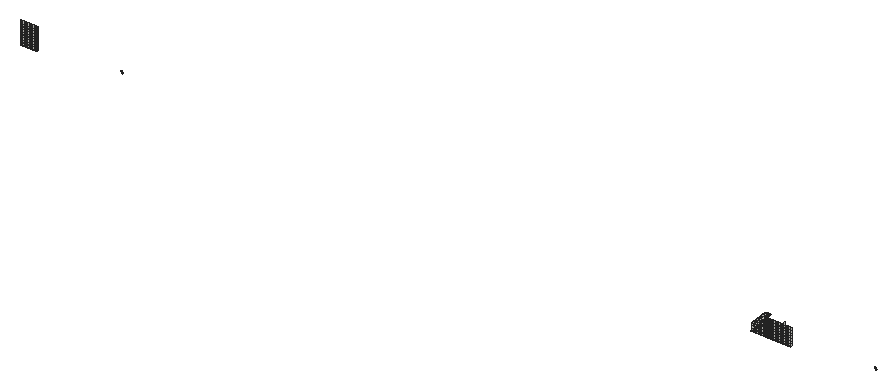
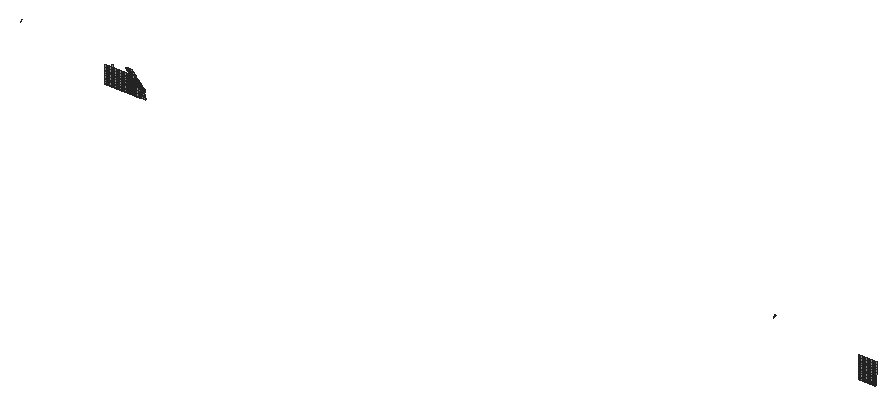
# SketchUp Ruby script. Lengths in inches.
U = 1.inch
M = Sketchup.active_model
def pt(a) = Geom::Point3d.new(a.map { |v| v * U })
def face(e, loops, mat)
  f = e.add_face(loops[0].map { |a| pt(a) })
  loops[1..].each { |l| e.add_face(l.map { |a| pt(a) }).erase! }
  f.material = f.back_material = mat if mat
  f
end
# faces: each face lists its corners as indices into pts; further lists are holes
def faces(e, pts, list, mat = nil) = list.each { |f| face(e, (f[0].is_a?(Array) ? f : [f]).map { |l| l.map { |i| pts[i] } }, mat) }
# xy, xz, yz: faces in a plane at the given z, y or x. An outline is a flat list of corners, or four numbers for a rectangle; further outlines are holes
def ring(l) = l.size == 4 ? [[l[0], l[1]], [l[2], l[1]], [l[2], l[3]], [l[0], l[3]]] : l.each_slice(2).to_a
def flat(e, list, mat, &to3) = list.each { |f| face(e, (f[0].is_a?(Array) ? f : [f]).map { |l| ring(l).map { |u, v| to3.(u, v) } }, mat) }
def xy(e, z, list, mat = nil) = flat(e, list, mat) { |x, y| [x, y, z] }
def xz(e, y, list, mat = nil) = flat(e, list, mat) { |x, z| [x, y, z] }
def yz(e, x, list, mat = nil) = flat(e, list, mat) { |y, z| [x, y, z] }
def lines(e, pts, list) = list.each { |a, b| e.add_line(pt(pts[a]), pt(pts[b])) }
# prism: a flat outline (further loops are holes) pulled along v
def prism(e, loops, v, mat = nil)
  f = face(e, loops, mat); d = Geom::Vector3d.new(v.map { |x| x * U })
  f.pushpull(f.normal.samedirection?(d) ? d.length : -d.length)
end
def box(e, o, s, mat = nil) = prism(e, [[o, [o[0] + s[0], o[1], o[2]], [o[0] + s[0], o[1] + s[1], o[2]], [o[0], o[1] + s[1], o[2]]]], [0, 0, s[2]], mat)
def at(x, y, z, deg = 0) = Geom::Transformation.translation(pt([x, y, z])) * Geom::Transformation.rotation(ORIGIN, Z_AXIS, deg.degrees)
def axes(o, x, y, z) = Geom::Transformation.new([*x, 0, *y, 0, *z, 0, *pt(o).to_a, 1])
def part(name) = M.definitions.add(name)
# library, detail: a bought-in or finely detailed component or shape, given as its bounding box
def library(name, o, s) = part(name).tap { |d| box(d.entities, o, s) }
def detail(e, o, s) = box(e.add_group.entities, o, s)
def put(e, d, t, mat = nil) = e.add_instance(d, t).tap { |i| i.material = mat if mat }
def group(e, t, mat = nil) = e.add_group.tap { |g| g.transformation = t; g.material = mat if mat }.entities
root = M.entities
M.materials.add("[Color M06]").color = [79, 71, 84]
xy(root,341.65,[[1366.25,480.14,1368.57,480.77],[1369.17,480.14,1371.48,480.77],[1372.08,480.14,1374.39,480.77],[1374.99,480.14,1377.3,480.77],[1377.9,480.14,1380.22,480.77],
  [1380.81,480.14,1383.13,480.77],[1383.73,480.14,1386.04,480.77],[2225.11,480.14,2225.91,480.77],[2226.51,480.14,2228.82,480.77],[2229.42,480.14,2231.73,480.77],
  [2232.33,480.14,2234.65,480.77],[2235.25,480.14,2237.56,480.77],[2238.16,480.14,2240.47,480.77],[2241.07,480.14,2243.38,480.77],[2243.98,480.14,2246.29,480.77],
  [2246.89,480.14,2249.21,480.77],[2249.81,480.14,2252.12,480.77],[2252.72,480.14,2255.03,480.77],[2255.63,480.14,2257.94,480.77],[2258.54,480.14,2260.86,480.77],
  [2261.45,480.14,2263.77,480.77],[2264.37,480.14,2266.68,480.77],[2267.28,480.14,2269.59,480.77],[2270.19,480.14,2272.5,480.77]])
xy(root,342.15,[[1366.25,480.14,1368.57,480.77],[1369.17,480.14,1371.48,480.77],[1372.08,480.14,1374.39,480.77],[1374.99,480.14,1377.3,480.77],[1377.9,480.14,1380.22,480.77],
  [1380.81,480.14,1383.13,480.77],[1383.73,480.14,1386.04,480.77],[2226.51,480.14,2228.82,480.77],[2229.42,480.14,2231.73,480.77],[2232.33,480.14,2234.65,480.77],
  [2235.25,480.14,2237.56,480.77],[2238.16,480.14,2240.47,480.77],[2241.07,480.14,2243.38,480.77],[2243.98,480.14,2246.29,480.77],[2246.89,480.14,2249.21,480.77],
  [2249.81,480.14,2252.12,480.77],[2252.72,480.14,2255.03,480.77],[2255.63,480.14,2257.94,480.77],[2258.54,480.14,2260.86,480.77],[2261.45,480.14,2263.77,480.77],
  [2264.37,480.14,2266.68,480.77],[2267.28,480.14,2269.59,480.77],[2270.19,480.14,2272.5,480.77]])
xy(root,344.46,[[1366.25,480.14,1368.57,480.77],[1369.17,480.14,1371.48,480.77],[1372.08,480.14,1374.39,480.77],[1374.99,480.14,1377.3,480.77],[1377.9,480.14,1380.22,480.77],
  [1380.81,480.14,1383.13,480.77],[2227.75,480.14,2228.82,480.77],[2229.42,480.14,2231.73,480.77],[2232.33,480.14,2234.65,480.77],[2235.25,480.14,2237.56,480.77],
  [2238.16,480.14,2240.47,480.77],[2241.07,480.14,2243.38,480.77],[2243.98,480.14,2246.29,480.77],[2246.89,480.14,2249.21,480.77],[2249.81,480.14,2252.12,480.77],
  [2252.72,480.14,2255.03,480.77],[2255.63,480.14,2257.94,480.77],[2258.54,480.14,2260.86,480.77],[2261.45,480.14,2263.77,480.77],[2264.37,480.14,2266.68,480.77],
  [2267.28,480.14,2269.59,480.77]])
xy(root,344.96,[[1366.25,480.14,1368.57,480.77],[1369.17,480.14,1371.48,480.77],[1372.08,480.14,1374.39,480.77],[1374.99,480.14,1377.3,480.77],[1377.9,480.14,1380.22,480.77],
  [1380.81,480.14,1383.13,480.77],[1383.73,480.14,1386.04,480.77],[2229.42,480.14,2231.73,480.77],[2232.33,480.14,2234.65,480.77],[2235.25,480.14,2237.56,480.77],
  [2238.16,480.14,2240.47,480.77],[2241.07,480.14,2243.38,480.77],[2243.98,480.14,2246.29,480.77],[2246.89,480.14,2249.21,480.77],[2249.81,480.14,2252.12,480.77],
  [2252.72,480.14,2255.03,480.77],[2255.63,480.14,2257.94,480.77],[2258.54,480.14,2260.86,480.77],[2261.45,480.14,2263.77,480.77],[2264.37,480.14,2266.68,480.77],
  [2267.28,480.14,2269.59,480.77],[2270.19,480.14,2272.5,480.77]])
xy(root,347.27,[[1366.25,480.14,1368.57,480.77],[1369.17,480.14,1371.48,480.77],[1372.08,480.14,1374.39,480.77],[1374.99,480.14,1377.3,480.77],[1377.9,480.14,1380.22,480.77],
  [1380.81,480.14,1383.13,480.77],[1383.73,480.14,1386.04,480.77],[2230.38,480.14,2231.73,480.77],[2232.33,480.14,2234.65,480.77],[2235.25,480.14,2237.56,480.77],
  [2238.16,480.14,2240.47,480.77],[2241.07,480.14,2243.38,480.77],[2243.98,480.14,2246.29,480.77],[2246.89,480.14,2249.21,480.77],[2249.81,480.14,2252.12,480.77],
  [2252.72,480.14,2255.03,480.77],[2255.63,480.14,2257.94,480.77],[2258.54,480.14,2260.86,480.77],[2261.45,480.14,2263.77,480.77],[2264.37,480.14,2266.68,480.77],
  [2267.28,480.14,2269.59,480.77],[2270.19,480.14,2272.5,480.77]])
xy(root,347.77,[[1366.25,480.14,1368.57,480.77],[1369.17,480.14,1371.48,480.77],[1372.08,480.14,1374.39,480.77],[1374.99,480.14,1377.3,480.77],[1377.9,480.14,1380.22,480.77],
  [1380.81,480.14,1383.13,480.77],[1383.73,480.14,1386.04,480.77],[2232.33,480.14,2234.65,480.77],[2235.25,480.14,2237.56,480.77],[2238.16,480.14,2240.47,480.77],
  [2241.07,480.14,2243.38,480.77],[2243.98,480.14,2246.29,480.77],[2246.89,480.14,2249.21,480.77],[2249.81,480.14,2252.12,480.77],[2252.72,480.14,2255.03,480.77],
  [2255.63,480.14,2257.94,480.77],[2258.54,480.14,2260.86,480.77],[2261.45,480.14,2263.77,480.77],[2264.37,480.14,2266.68,480.77],[2267.28,480.14,2269.59,480.77],
  [2270.19,480.14,2272.5,480.77]])
xy(root,350.09,[[1366.25,480.14,1368.57,480.77],[1369.17,480.14,1371.48,480.77],[1372.08,480.14,1374.39,480.77],[1374.99,480.14,1377.3,480.77],[1377.9,480.14,1380.22,480.77],
  [1380.81,480.14,1383.13,480.77],[1383.73,480.14,1386.04,480.77],[2233.02,480.14,2234.65,480.77],[2235.25,480.14,2237.56,480.77],[2238.16,480.14,2240.47,480.77],
  [2241.07,480.14,2243.38,480.77],[2243.98,480.14,2246.29,480.77],[2246.89,480.14,2249.21,480.77],[2249.81,480.14,2252.12,480.77],[2252.72,480.14,2255.03,480.77],
  [2255.63,480.14,2257.94,480.77],[2258.54,480.14,2260.86,480.77],[2261.45,480.14,2263.77,480.77],[2264.37,480.14,2266.68,480.77],[2267.28,480.14,2269.59,480.77],
  [2270.19,480.14,2272.5,480.77]])
xy(root,350.59,[[1366.25,480.14,1368.57,480.77],[1369.17,480.14,1371.48,480.77],[1372.08,480.14,1374.39,480.77],[1374.99,480.14,1377.3,480.77],[1377.9,480.14,1380.22,480.77],
  [1380.81,480.14,1383.13,480.77],[1383.73,480.14,1386.04,480.77],[2235.25,480.14,2237.56,480.77],[2238.16,480.14,2240.47,480.77],[2241.07,480.14,2243.38,480.77],
  [2243.98,480.14,2246.29,480.77],[2246.89,480.14,2249.21,480.77],[2249.81,480.14,2252.12,480.77],[2252.72,480.14,2255.03,480.77],[2255.63,480.14,2257.94,480.77],
  [2258.54,480.14,2260.86,480.77],[2261.45,480.14,2263.77,480.77],[2264.37,480.14,2266.68,480.77],[2267.28,480.14,2269.59,480.77],[2270.19,480.14,2272.5,480.77]])
xy(root,352.9,[[1366.25,480.14,1368.57,480.77],[1369.17,480.14,1371.48,480.77],[1372.08,480.14,1374.39,480.77],[1374.99,480.14,1377.3,480.77],[1377.9,480.14,1380.22,480.77],
  [1380.81,480.14,1383.13,480.77],[1383.73,480.14,1386.04,480.77],[2235.65,480.14,2237.56,480.77],[2238.16,480.14,2240.47,480.77],[2241.07,480.14,2243.38,480.77],
  [2243.98,480.14,2246.29,480.77],[2246.89,480.14,2249.21,480.77],[2249.81,480.14,2252.12,480.77],[2252.72,480.14,2255.03,480.77],[2255.63,480.14,2257.94,480.77],
  [2258.54,480.14,2260.86,480.77],[2261.45,480.14,2263.77,480.77],[2264.37,480.14,2266.68,480.77],[2267.28,480.14,2269.59,480.77],[2270.19,480.14,2272.5,480.77]])
xy(root,353.4,[[1366.25,480.14,1368.57,480.77],[1369.17,480.14,1371.48,480.77],[1372.08,480.14,1374.39,480.77],[1374.99,480.14,1377.3,480.77],[1377.9,480.14,1380.22,480.77],
  [1380.81,480.14,1383.13,480.77],[1383.73,480.14,1386.04,480.77],[2236.12,480.14,2237.56,480.77],[2238.16,480.14,2240.47,480.77],[2241.07,480.14,2243.38,480.77],
  [2243.98,480.14,2246.29,480.77],[2246.89,480.14,2249.21,480.77],[2249.81,480.14,2252.12,480.77],[2252.72,480.14,2255.03,480.77],[2255.63,480.14,2257.94,480.77],
  [2258.54,480.14,2260.86,480.77],[2261.45,480.14,2263.77,480.77],[2264.37,480.14,2266.68,480.77],[2267.28,480.14,2269.59,480.77],[2270.19,480.14,2272.5,480.77]])
xy(root,355.71,[[1366.25,480.14,1368.57,480.77],[1369.17,480.14,1371.48,480.77],[1372.08,480.14,1374.39,480.77],[1374.99,480.14,1377.3,480.77],[1377.9,480.14,1380.22,480.77],
  [1380.81,480.14,1383.13,480.77],[1383.73,480.14,1386.04,480.77],[2238.29,480.14,2240.47,480.77],[2241.07,480.14,2243.38,480.77],[2243.98,480.14,2246.29,480.77],
  [2246.89,480.14,2249.21,480.77],[2249.81,480.14,2252.12,480.77],[2252.72,480.14,2255.03,480.77],[2255.63,480.14,2257.94,480.77],[2258.54,480.14,2260.86,480.77],
  [2261.45,480.14,2263.77,480.77],[2264.37,480.14,2266.68,480.77],[2267.28,480.14,2269.59,480.77],[2270.19,480.14,2272.5,480.77]])
xy(root,356.21,[[1366.25,480.14,1368.57,480.77],[1369.17,480.14,1371.48,480.77],[1372.08,480.14,1374.39,480.77],[1374.99,480.14,1377.3,480.77],[1377.9,480.14,1380.22,480.77],
  [1380.81,480.14,1383.13,480.77],[1383.73,480.14,1386.04,480.77],[2238.76,480.14,2240.47,480.77],[2241.07,480.14,2243.38,480.77],[2243.98,480.14,2246.29,480.77],
  [2246.89,480.14,2249.21,480.77],[2249.81,480.14,2252.12,480.77],[2252.72,480.14,2255.03,480.77],[2255.63,480.14,2257.94,480.77],[2258.54,480.14,2260.86,480.77],
  [2261.45,480.14,2263.77,480.77],[2264.37,480.14,2266.68,480.77],[2267.28,480.14,2269.59,480.77],[2270.19,480.14,2272.5,480.77]])
xy(root,358.52,[[1366.25,480.14,1368.57,480.77],[1369.17,480.14,1371.48,480.77],[1372.08,480.14,1374.39,480.77],[1374.99,480.14,1377.3,480.77],[1377.9,480.14,1380.22,480.77],
  [1380.81,480.14,1383.13,480.77],[1383.73,480.14,1386.04,480.77],[2241.07,480.14,2243.38,480.77],[2243.98,480.14,2246.29,480.77],[2246.89,480.14,2249.21,480.77],
  [2249.81,480.14,2252.12,480.77],[2252.72,480.14,2255.03,480.77],[2255.63,480.14,2257.94,480.77],[2258.54,480.14,2260.86,480.77],[2261.45,480.14,2263.77,480.77],
  [2264.37,480.14,2266.68,480.77],[2267.28,480.14,2269.59,480.77],[2270.19,480.14,2272.5,480.77]])
xy(root,359.02,[[1366.25,480.14,1368.57,480.77],[1369.17,480.14,1371.48,480.77],[1372.08,480.14,1374.39,480.77],[1374.99,480.14,1377.3,480.77],[1377.9,480.14,1380.22,480.77],
  [1380.81,480.14,1383.13,480.77],[1383.73,480.14,1386.04,480.77],[2241.4,480.14,2243.38,480.77],[2243.98,480.14,2246.29,480.77],[2246.89,480.14,2249.21,480.77],
  [2249.81,480.14,2252.12,480.77],[2252.72,480.14,2255.03,480.77],[2255.63,480.14,2257.94,480.77],[2258.54,480.14,2260.86,480.77],[2261.45,480.14,2263.77,480.77],
  [2264.37,480.14,2266.68,480.77],[2267.28,480.14,2269.59,480.77],[2270.19,480.14,2272.5,480.77]])
xy(root,361.34,[[1366.25,480.14,1368.57,480.77],[1369.17,480.14,1371.48,480.77],[1372.08,480.14,1374.39,480.77],[1374.99,480.14,1377.3,480.77],[1377.9,480.14,1380.22,480.77],
  [1380.81,480.14,1383.13,480.77],[1383.73,480.14,1386.04,480.77],[2243.98,480.14,2246.29,480.77],[2246.89,480.14,2249.21,480.77],[2249.81,480.14,2252.12,480.77],
  [2252.72,480.14,2255.03,480.77],[2255.63,480.14,2257.94,480.77],[2258.54,480.14,2260.86,480.77],[2261.45,480.14,2263.77,480.77],[2264.37,480.14,2266.68,480.77],
  [2267.28,480.14,2269.59,480.77],[2270.19,480.14,2272.5,480.77]])
xy(root,361.84,[[1366.25,480.14,1368.57,480.77],[1369.17,480.14,1371.48,480.77],[1372.08,480.14,1374.39,480.77],[1374.99,480.14,1377.3,480.77],[1377.9,480.14,1380.22,480.77],
  [1380.81,480.14,1383.13,480.77],[1383.73,480.14,1386.04,480.77]])
xy(root,364.15,[[1366.25,480.14,1368.57,480.77],[1369.17,480.14,1371.48,480.77],[1372.08,480.14,1374.39,480.77],[1374.99,480.14,1377.3,480.77],[1377.9,480.14,1380.22,480.77],
  [1380.81,480.14,1383.13,480.77],[1383.73,480.14,1386.04,480.77]])
xy(root,364.65,[[1366.25,480.14,1368.57,480.77],[1369.17,480.14,1371.48,480.77],[1372.08,480.14,1374.39,480.77],[1374.99,480.14,1377.3,480.77],[1377.9,480.14,1380.22,480.77],
  [1380.81,480.14,1383.13,480.77],[1383.73,480.14,1386.04,480.77]])
xz(root,467.1875,[[1496.3,361.83,1496.67,362.07,1494.98,364.71,1494.61,364.48],[2382.77,361.83,2383.14,362.07,2381.44,364.71,2381.07,364.48]],"[Color M06]")
xz(root,480.14,[[2226.51,343.14,2227.75,344.46,2226.51,344.46],[2226.51,344.96,2228.21,344.96,2228.82,345.61,2228.82,347.27,2227.75,347.27,2226.51,345.96],[2228.21,344.96,2228.82,344.96,2228.82,345.61],[2229.42,346.25,2230.38,347.27,2229.42,347.27],[2226.51,347.77,2226.52,347.77,2228.69,350.09,2227.75,350.09,2226.51,348.77],
  [2226.52,347.77,2228.21,347.77,2228.82,348.42,2228.82,350.09,2228.69,350.09],[2229.42,347.77,2230.85,347.77,2231.73,348.72,2231.73,350.09,2230.38,350.09,2229.42,349.0625],[2230.85,347.77,2231.73,347.77,2231.73,348.72],[2232.33,349.36,2233.02,350.09,2232.33,350.09],[2226.52,350.59,2226.57,350.59,2228.75,352.9,2228.69,352.9],
  [2226.57,350.59,2228.21,350.59,2228.82,351.24,2228.82,352.9,2228.75,352.9],[2228.21,350.59,2228.82,350.59,2228.82,351.24],[2229.42,350.59,2230.85,350.59,2231.73,351.53,2231.73,352.9,2231.34,352.9,2229.42,350.86],[2232.33,350.59,2233.49,350.59,2234.65,351.82,2234.65,352.9,2233.02,352.9,2232.33,352.17],[2233.49,350.59,2234.65,350.59,2234.65,351.82],
  [2229.42,350.86,2231.34,352.9,2230.38,352.9,2229.42,351.875],[2235.25,352.46,2235.65,352.9,2235.25,352.9],[2229.42,353.4,2230.85,353.4,2231.73,354.34,2231.73,355.71,2231.4,355.71,2229.42,353.62],[2230.85,353.4,2231.73,353.4,2231.73,354.34],[2232.33,353.4,2233.49,353.4,2234.65,354.64,2234.65,355.71,2233.99,355.71,2232.33,353.95],
  [2235.25,353.4,2236.12,353.4,2237.56,354.93,2237.56,355.71,2235.65,355.71,2235.25,355.28],[2229.42,353.62,2231.4,355.71,2231.34,355.71,2229.42,353.67],[2232.33,353.95,2233.99,355.71,2233.02,355.71,2232.33,354.98],[2238.16,355.57,2238.29,355.71,2238.16,355.71],[2232.33,356.21,2233.49,356.21,2234.65,357.45,2234.65,358.52,2234.04,358.52,2232.33,356.71],
  [2234.46,356.21,2234.65,356.21,2234.65,356.41],[2235.25,356.21,2236.12,356.21,2237.56,357.74,2237.56,358.52,2236.64,358.52,2235.25,357.05],[2238.16,356.21,2238.76,356.21,2240.47,358.04,2240.47,358.52,2238.29,358.52,2238.16,358.38],[2232.33,356.71,2234.04,358.52,2233.99,358.52,2232.33,356.77],[2235.25,357.05,2236.64,358.52,2235.65,358.52,2235.25,358.09],
  [2238.16,358.38,2238.29,358.52,2238.16,358.52],[2234.51,359.02,2234.65,359.02,2234.65,359.17],[2235.25,359.02,2236.12,359.02,2237.56,360.56,2237.56,361.34,2236.69,361.34,2235.25,359.8],[2237.11,359.02,2237.56,359.02,2237.56,359.5],[2238.16,359.02,2240.47,359.02,2240.47,361.34,2239.28,361.34,2238.16,360.14],
  [2241.07,359.02,2241.4,359.02,2243.38,361.14,2243.38,361.34,2241.07,361.34],[2235.25,359.8,2236.69,361.34,2236.64,361.34,2235.25,359.86],[2238.16,361.2,2238.29,361.34,2238.16,361.34],[2237.16,361.84,2237.56,361.84,2237.56,362.26],[2238.16,361.84,2239.75,361.84,2240.47,362.6,2240.47,364.15,2239.34,364.15,2238.16,362.9],
  [2239.75,361.84,2240.47,361.84,2240.47,362.6],[2241.07,361.84,2241.4,361.84,2243.38,363.96,2243.38,364.15,2241.93,364.15,2241.07,363.23],[2241.4,361.84,2243.38,361.84,2243.38,363.96],[2241.07,363.23,2241.93,364.15,2241.07,364.15],[2239.81,364.65,2240.47,364.65,2240.47,365.35],
  [2241.07,364.65,2241.4,364.65,2243.38,366.77,2243.38,366.96,2241.99,366.96,2241.07,365.99],[2241.4,364.65,2242.4,364.65,2243.38,365.69,2243.38,366.77],[2242.4,364.65,2243.38,364.65,2243.38,365.69],[2243.98,364.65,2244.03,364.65,2246.2,366.96,2244.58,366.96,2243.98,366.33],[2244.03,364.65,2246.29,364.65,2246.29,366.96,2246.2,366.96]])
xz(root,480.14,[[2243.98,361.84,2244.03,361.84,2246.2,364.15,2243.98,364.15],[2246.89,364.89,2248.83,366.96,2246.89,366.96]],"[Color M06]")
yz(root,1365.65,[[480.14,353.4,480.77,355.71],[480.14,356.21,480.77,358.52],[480.14,359.02,480.77,361.34],[480.14,361.84,480.77,364.15],[480.14,364.65,480.77,366.96]])
yz(root,1366.25,[[480.14,342.15,480.77,344.46],[480.14,344.96,480.77,347.27],[480.14,347.77,480.77,350.09],[480.14,350.59,480.77,352.9],[480.14,353.4,480.77,355.71],
  [480.14,356.21,480.77,358.52],[480.14,359.02,480.77,361.34],[480.14,361.84,480.77,364.15],[480.14,364.65,480.77,366.96]])
yz(root,1368.57,[[480.14,342.15,480.77,344.46],[480.14,344.96,480.77,347.27],[480.14,347.77,480.77,350.09],[480.14,350.59,480.77,352.9],[480.14,353.4,480.77,355.71],
  [480.14,356.21,480.77,358.52],[480.14,359.02,480.77,361.34],[480.14,361.84,480.77,364.15],[480.14,364.65,480.77,366.96]])
yz(root,1369.17,[[480.14,342.15,480.77,344.46],[480.14,344.96,480.77,347.27],[480.14,347.77,480.77,350.09],[480.14,350.59,480.77,352.9],[480.14,353.4,480.77,355.71],
  [480.14,356.21,480.77,358.52],[480.14,359.02,480.77,361.34],[480.14,361.84,480.77,364.15],[480.14,364.65,480.77,366.96]])
yz(root,1371.48,[[480.14,342.15,480.77,344.46],[480.14,344.96,480.77,347.27],[480.14,347.77,480.77,350.09],[480.14,350.59,480.77,352.9],[480.14,353.4,480.77,355.71],
  [480.14,356.21,480.77,358.52],[480.14,359.02,480.77,361.34],[480.14,361.84,480.77,364.15],[480.14,364.65,480.77,366.96]])
yz(root,1372.08,[[480.14,342.15,480.77,344.46],[480.14,344.96,480.77,347.27],[480.14,347.77,480.77,350.09],[480.14,350.59,480.77,352.9],[480.14,353.4,480.77,355.71],
  [480.14,356.21,480.77,358.52],[480.14,359.02,480.77,361.34],[480.14,361.84,480.77,364.15],[480.14,364.65,480.77,366.96]])
yz(root,1374.39,[[480.14,342.15,480.77,344.46],[480.14,344.96,480.77,347.27],[480.14,347.77,480.77,350.09],[480.14,350.59,480.77,352.9],[480.14,353.4,480.77,355.71],
  [480.14,356.21,480.77,358.52],[480.14,359.02,480.77,361.34],[480.14,361.84,480.77,364.15],[480.14,364.65,480.77,366.96]])
yz(root,1374.99,[[480.14,342.15,480.77,344.46],[480.14,344.96,480.77,347.27],[480.14,347.77,480.77,350.09],[480.14,350.59,480.77,352.9],[480.14,353.4,480.77,355.71],
  [480.14,356.21,480.77,358.52],[480.14,359.02,480.77,361.34],[480.14,361.84,480.77,364.15],[480.14,364.65,480.77,366.96]])
yz(root,1377.3,[[480.14,342.15,480.77,344.46],[480.14,344.96,480.77,347.27],[480.14,347.77,480.77,350.09],[480.14,350.59,480.77,352.9],[480.14,353.4,480.77,355.71],
  [480.14,356.21,480.77,358.52],[480.14,359.02,480.77,361.34],[480.14,361.84,480.77,364.15],[480.14,364.65,480.77,366.96]])
yz(root,1377.9,[[480.14,342.15,480.77,344.46],[480.14,344.96,480.77,347.27],[480.14,347.77,480.77,350.09],[480.14,350.59,480.77,352.9],[480.14,353.4,480.77,355.71],
  [480.14,356.21,480.77,358.52],[480.14,359.02,480.77,361.34],[480.14,361.84,480.77,364.15],[480.14,364.65,480.77,366.96]])
yz(root,1380.22,[[480.14,342.15,480.77,344.46],[480.14,344.96,480.77,347.27],[480.14,347.77,480.77,350.09],[480.14,350.59,480.77,352.9],[480.14,353.4,480.77,355.71],
  [480.14,356.21,480.77,358.52],[480.14,359.02,480.77,361.34],[480.14,361.84,480.77,364.15],[480.14,364.65,480.77,366.96]])
yz(root,1380.81,[[480.14,342.15,480.77,344.46],[480.14,344.96,480.77,347.27],[480.14,347.77,480.77,350.09],[480.14,350.59,480.77,352.9],[480.14,353.4,480.77,355.71],
  [480.14,356.21,480.77,358.52],[480.14,359.02,480.77,361.34],[480.14,361.84,480.77,364.15],[480.14,364.65,480.77,366.96]])
yz(root,1383.13,[[480.14,342.15,480.77,344.46],[480.14,344.96,480.77,347.27],[480.14,347.77,480.77,350.09],[480.14,350.59,480.77,352.9],[480.14,353.4,480.77,355.71],
  [480.14,356.21,480.77,358.52],[480.14,359.02,480.77,361.34],[480.14,361.84,480.77,364.15],[480.14,364.65,480.77,366.96]])
yz(root,1383.73,[[480.14,342.15,480.77,344.46],[480.14,344.96,480.77,347.27],[480.14,347.77,480.77,350.09],[480.14,350.59,480.77,352.9],[480.14,353.4,480.77,355.71],
  [480.14,356.21,480.77,358.52],[480.14,359.02,480.77,361.34],[480.14,361.84,480.77,364.15],[480.14,364.65,480.77,366.96]])
yz(root,1386.04,[[480.14,342.15,480.77,344.46],[480.14,344.96,480.77,347.27],[480.14,347.77,480.77,350.09],[480.14,350.59,480.77,352.9],[480.14,353.4,480.77,355.71],
  [480.14,356.21,480.77,358.52],[480.14,359.02,480.77,361.34],[480.14,361.84,480.77,364.15],[480.14,364.65,480.77,366.96]])
yz(root,2226.51,[[480.14,342.15,480.77,343.14]])
yz(root,2228.82,[[480.14,342.15,480.77,344.46]])
yz(root,2229.42,[[480.14,342.15,480.77,344.46],[480.14,344.96,480.77,346.25]])
yz(root,2231.73,[[480.14,342.15,480.77,344.46],[480.14,344.96,480.77,347.27]])
yz(root,2232.33,[[480.14,342.15,480.77,344.46],[480.14,344.96,480.77,347.27],[480.14,347.77,480.77,349.36]])
yz(root,2234.65,[[480.14,342.15,480.77,344.46],[480.14,344.96,480.77,347.27],[480.14,347.77,480.77,350.09]])
yz(root,2235.25,[[480.14,342.15,480.77,344.46],[480.14,344.96,480.77,347.27],[480.14,347.77,480.77,350.09],[480.14,350.59,480.77,352.46]])
yz(root,2237.56,[[480.14,342.15,480.77,344.46],[480.14,344.96,480.77,347.27],[480.14,347.77,480.77,350.09],[480.14,350.59,480.77,352.9],[480.14,353.4,480.77,354.93]])
yz(root,2238.16,[[480.14,342.15,480.77,344.46],[480.14,344.96,480.77,347.27],[480.14,347.77,480.77,350.09],[480.14,350.59,480.77,352.9],[480.14,353.4,480.77,355.57]])
yz(root,2240.47,[[480.14,342.15,480.77,344.46],[480.14,344.96,480.77,347.27],[480.14,347.77,480.77,350.09],[480.14,350.59,480.77,352.9],[480.14,353.4,480.77,355.71],
  [480.14,356.21,480.77,358.04]])
yz(root,2241.07,[[480.14,342.15,480.77,344.46],[480.14,344.96,480.77,347.27],[480.14,347.77,480.77,350.09],[480.14,350.59,480.77,352.9],[480.14,353.4,480.77,355.71],
  [480.14,356.21,480.77,358.52]])
yz(root,2243.38,[[480.14,342.15,480.77,344.46],[480.14,344.96,480.77,347.27],[480.14,347.77,480.77,350.09],[480.14,350.59,480.77,352.9],[480.14,353.4,480.77,355.71],
  [480.14,356.21,480.77,358.52],[480.14,359.02,480.77,361.14]])
yz(root,2243.98,[[480.14,342.15,480.77,344.46],[480.14,344.96,480.77,347.27],[480.14,347.77,480.77,350.09],[480.14,350.59,480.77,352.9],[480.14,353.4,480.77,355.71],
  [480.14,356.21,480.77,358.52],[480.14,359.02,480.77,361.34]])
yz(root,2246.29,[[480.14,342.15,480.77,344.46],[480.14,344.96,480.77,347.27],[480.14,347.77,480.77,350.09],[480.14,350.59,480.77,352.9],[480.14,353.4,480.77,355.71],
  [480.14,356.21,480.77,358.52],[480.14,359.02,480.77,361.34]])
yz(root,2246.89,[[480.14,342.15,480.77,344.46],[480.14,344.96,480.77,347.27],[480.14,347.77,480.77,350.09],[480.14,350.59,480.77,352.9],[480.14,353.4,480.77,355.71],
  [480.14,356.21,480.77,358.52],[480.14,359.02,480.77,361.34]])
yz(root,2249.21,[[480.14,342.15,480.77,344.46],[480.14,344.96,480.77,347.27],[480.14,347.77,480.77,350.09],[480.14,350.59,480.77,352.9],[480.14,353.4,480.77,355.71],
  [480.14,356.21,480.77,358.52],[480.14,359.02,480.77,361.34]])
yz(root,2249.81,[[480.14,342.15,480.77,344.46],[480.14,344.96,480.77,347.27],[480.14,347.77,480.77,350.09],[480.14,350.59,480.77,352.9],[480.14,353.4,480.77,355.71],
  [480.14,356.21,480.77,358.52],[480.14,359.02,480.77,361.34]])
yz(root,2252.12,[[480.14,342.15,480.77,344.46],[480.14,344.96,480.77,347.27],[480.14,347.77,480.77,350.09],[480.14,350.59,480.77,352.9],[480.14,353.4,480.77,355.71],
  [480.14,356.21,480.77,358.52],[480.14,359.02,480.77,361.34]])
yz(root,2252.72,[[480.14,342.15,480.77,344.46],[480.14,344.96,480.77,347.27],[480.14,347.77,480.77,350.09],[480.14,350.59,480.77,352.9],[480.14,353.4,480.77,355.71],
  [480.14,356.21,480.77,358.52],[480.14,359.02,480.77,361.34]])
yz(root,2255.03,[[480.14,342.15,480.77,344.46],[480.14,344.96,480.77,347.27],[480.14,347.77,480.77,350.09],[480.14,350.59,480.77,352.9],[480.14,353.4,480.77,355.71],
  [480.14,356.21,480.77,358.52],[480.14,359.02,480.77,361.34]])
yz(root,2255.63,[[480.14,342.15,480.77,344.46],[480.14,344.96,480.77,347.27],[480.14,347.77,480.77,350.09],[480.14,350.59,480.77,352.9],[480.14,353.4,480.77,355.71],
  [480.14,356.21,480.77,358.52],[480.14,359.02,480.77,361.34]])
yz(root,2257.94,[[480.14,342.15,480.77,344.46],[480.14,344.96,480.77,347.27],[480.14,347.77,480.77,350.09],[480.14,350.59,480.77,352.9],[480.14,353.4,480.77,355.71],
  [480.14,356.21,480.77,358.52],[480.14,359.02,480.77,361.34]])
yz(root,2258.54,[[480.14,342.15,480.77,344.46],[480.14,344.96,480.77,347.27],[480.14,347.77,480.77,350.09],[480.14,350.59,480.77,352.9],[480.14,353.4,480.77,355.71],
  [480.14,356.21,480.77,358.52],[480.14,359.02,480.77,361.34]])
yz(root,2260.86,[[480.14,342.15,480.77,344.46],[480.14,344.96,480.77,347.27],[480.14,347.77,480.77,350.09],[480.14,350.59,480.77,352.9],[480.14,353.4,480.77,355.71],
  [480.14,356.21,480.77,358.52],[480.14,359.02,480.77,361.34]])
yz(root,2261.45,[[480.14,342.15,480.77,344.46],[480.14,344.96,480.77,347.27],[480.14,347.77,480.77,350.09],[480.14,350.59,480.77,352.9],[480.14,353.4,480.77,355.71],
  [480.14,356.21,480.77,358.52],[480.14,359.02,480.77,361.34]])
yz(root,2263.77,[[480.14,342.15,480.77,344.46],[480.14,344.96,480.77,347.27],[480.14,347.77,480.77,350.09],[480.14,350.59,480.77,352.9],[480.14,353.4,480.77,355.71],
  [480.14,356.21,480.77,358.52],[480.14,359.02,480.77,361.34]])
yz(root,2264.37,[[480.14,342.15,480.77,344.46],[480.14,344.96,480.77,347.27],[480.14,347.77,480.77,350.09],[480.14,350.59,480.77,352.9],[480.14,353.4,480.77,355.71],
  [480.14,356.21,480.77,358.52],[480.14,359.02,480.77,361.34],[480.14,361.84,480.77,364.15]])
yz(root,2266.68,[[480.14,342.15,480.77,344.46],[480.14,344.96,480.77,347.27],[480.14,347.77,480.77,350.09],[480.14,350.59,480.77,352.9],[480.14,353.4,480.77,355.71],
  [480.14,356.21,480.77,358.52],[480.14,359.02,480.77,361.34]])
yz(root,2267.28,[[480.14,342.15,480.77,344.46],[480.14,344.96,480.77,347.27],[480.14,347.77,480.77,350.09],[480.14,350.59,480.77,352.9],[480.14,353.4,480.77,355.71],
  [480.14,356.21,480.77,358.52],[480.14,359.02,480.77,361.34]])
yz(root,2269.59,[[480.14,342.15,480.77,344.46],[480.14,344.96,480.77,347.27],[480.14,347.77,480.77,350.09],[480.14,350.59,480.77,352.9],[480.14,353.4,480.77,355.71],
  [480.14,356.21,480.77,358.52],[480.14,359.02,480.77,361.34]])
yz(root,2270.19,[[480.14,342.15,480.77,344.46],[480.14,344.96,480.77,347.27],[480.14,347.77,480.77,350.09],[480.14,350.59,480.77,352.9],[480.14,353.4,480.77,355.71],
  [480.14,356.21,480.77,358.52],[480.14,359.02,480.77,361.34]])
yz(root,2272.5,[[480.14,342.15,480.77,344.46],[480.14,344.96,480.77,347.27],[480.14,347.77,480.77,350.09],[480.14,350.59,480.77,352.9],[480.14,353.4,480.77,355.71],
  [480.14,356.21,480.77,358.52],[480.14,359.02,480.77,361.34]])
p = [[2227.75,480.14,344.46],[2226.51,480.14,343.14],[2226.51,480.77,343.14],[2227.75,480.77,344.46],[2230.38,480.14,347.27],[2229.42,480.14,346.25],
  [2229.42,480.77,346.25],[2230.38,480.77,347.27],[2233.02,480.14,350.09],[2232.33,480.14,349.36],[2232.33,480.77,349.36],[2233.02,480.77,350.09],
  [2235.65,480.14,352.9],[2235.25,480.14,352.46],[2235.25,480.77,352.46],[2235.65,480.77,352.9],[2237.56,480.14,354.93],[2236.12,480.14,353.4],
  [2236.12,480.77,353.4],[2237.56,480.77,354.93],[2238.29,480.14,355.71],[2238.16,480.14,355.57],[2238.16,480.77,355.57],[2238.29,480.77,355.71],
  [2240.47,480.14,358.04],[2238.76,480.14,356.21],[2238.76,480.77,356.21],[2240.47,480.77,358.04],[2243.38,480.14,361.14],[2241.4,480.14,359.02],
  [2241.4,480.77,359.02],[2243.38,480.77,361.14],[2235.25,480.14,358.09],[2235.25,480.14,358.52],[2234.65,480.14,354.64],[2234.65,480.14,353.4],
  [2235.25,480.14,355.28],[2235.25,480.14,355.71],[2232.33,480.14,354.98],[2232.33,480.14,355.71],[2228.82,480.14,347.77],[2228.21,480.14,347.77],
  [2226.51,480.14,350.09],[2227.75,480.14,350.09],[2240.47,480.14,365.41],[2240.47,480.14,365.35],[2229.42,480.14,350.09],[2230.38,480.14,350.09],
  [2229.42,480.14,350.86],[2228.69,480.14,350.09],[2226.51,480.14,347.27],[2227.75,480.14,347.27],[2226.51,480.14,345.96],[2235.65,480.14,355.71],
  [2229.42,480.14,349.0625],[2228.82,480.14,348.42],[2232.33,480.14,352.9],[2233.02,480.14,352.9],[2226.51,480.14,348.77],[2229.42,480.14,352.9],
  [2230.38,480.14,352.9],[2229.42,480.14,351.875],[2231.73,480.14,351.53],[2231.73,480.14,350.59],[2226.52,480.14,350.59],[2226.51,480.14,350.59],
  [2230.85,480.14,350.59],[2232.33,480.14,352.17],[2233.49,480.14,353.4],[2235.65,480.14,358.52],[2232.33,480.14,353.95],[2231.34,480.14,352.9],
  [2233.02,480.14,355.71],[2234.51,480.14,361.84],[2234.46,480.14,361.84],[2239.28,480.14,364.15],[2239.34,480.14,364.15],[2238.16,480.14,362.9],
  [2238.16,480.14,364.15],[2241.07,480.14,363.23],[2240.47,480.14,362.6],[2239.75,480.14,361.84],[2239.28,480.14,361.34],[2237.16,480.14,361.84],
  [2237.11,480.14,361.84],[2239.81,480.14,364.65],[2239.75,480.14,364.65],[2235.25,480.14,357.05],[2234.65,480.14,356.41],[2234.46,480.14,356.21],
  [2233.99,480.14,355.71],[2237.56,480.14,356.21],[2236.12,480.14,356.21],[2233.49,480.14,356.21],[2234.65,480.14,359.22],[2234.65,480.14,359.17],
  [2237.56,480.14,360.56],[2237.56,480.14,359.5],[2238.29,480.14,361.34],[2242.4,480.14,364.65],[2241.93,480.14,364.15],[2238.16,480.14,360.14],
  [2237.11,480.14,359.02],[2236.12,480.14,359.02],[2236.64,480.14,358.52],[2234.51,480.14,359.02],[2234.46,480.14,359.02],[2238.16,480.14,361.2],
  [2243.98,480.14,366.33],[2243.38,480.14,365.69],[2237.56,480.14,357.74],[2234.65,480.14,357.45],[2231.73,480.14,356.21],[2230.85,480.14,356.21]]
faces(root,p,[[0,1,2,3],[4,5,6,7],[8,9,10,11],[12,13,14,15],[16,17,18,19],[20,21,22,23],[24,25,26,27],[28,29,30,31]])
lines(root,p,[[32,33],[34,35],[36,37],[38,39],[40,41],[42,43],[44,45],[46,47],[48,49],[50,51],[52,50],[37,53],
  [54,46],[55,40],[56,57],[58,42],[59,60],[61,59],[62,63],[64,65],[63,66],[67,56],[35,68],[33,69],
  [70,71],[39,72],[73,74],[75,76],[77,78],[79,80],[81,82],[83,84],[85,86],[87,88],[89,90],[91,92],
  [89,93],[94,95],[96,97],[98,82],[99,100],[101,97],[102,103],[102,104],[105,106],[101,107],[108,109],[110,91],
  [111,88],[112,113]])
